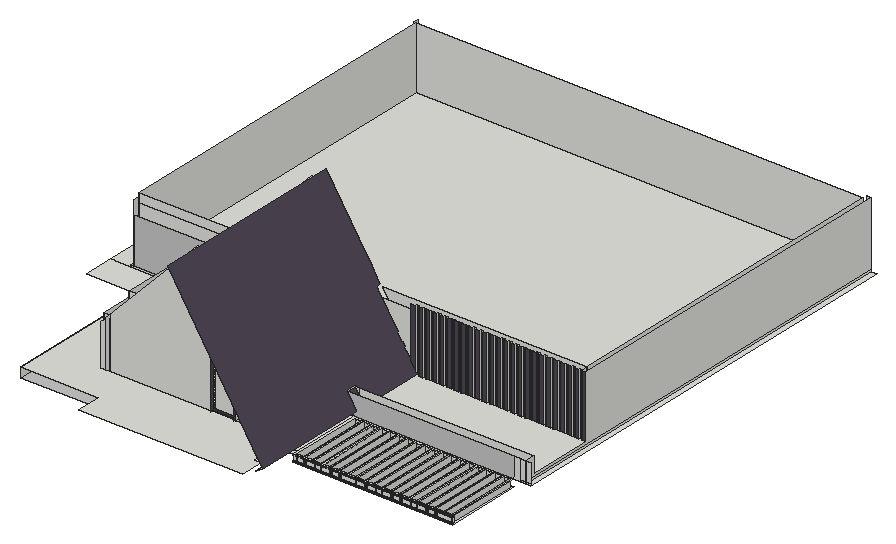
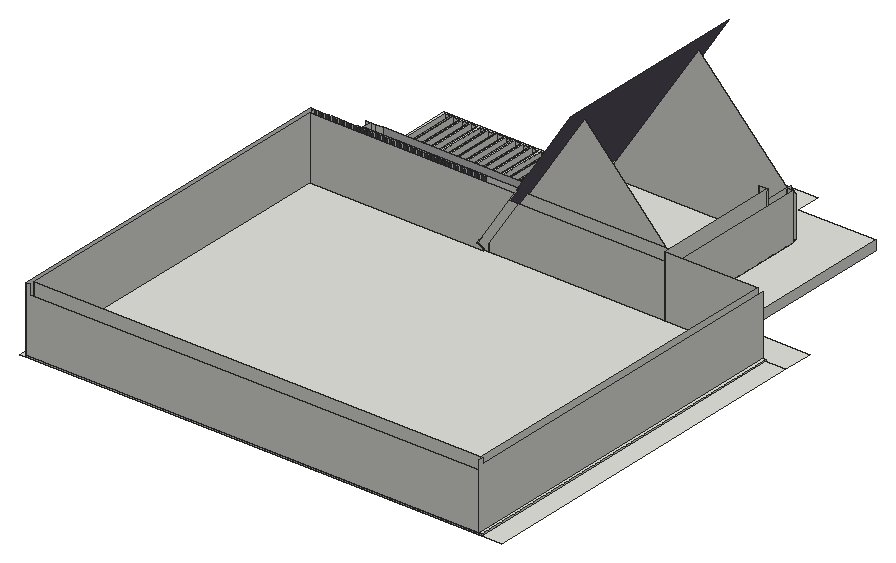
# SketchUp Ruby script. Lengths in inches.
U = 1.inch
M = Sketchup.active_model
def pt(a) = Geom::Point3d.new(a.map { |v| v * U })
def face(e, loops, mat)
  f = e.add_face(loops[0].map { |a| pt(a) })
  loops[1..].each { |l| e.add_face(l.map { |a| pt(a) }).erase! }
  f.material = f.back_material = mat if mat
  f
end
# faces: each face lists its corners as indices into pts; further lists are holes
def faces(e, pts, list, mat = nil) = list.each { |f| face(e, (f[0].is_a?(Array) ? f : [f]).map { |l| l.map { |i| pts[i] } }, mat) }
# xy, xz, yz: faces in a plane at the given z, y or x. An outline is a flat list of corners, or four numbers for a rectangle; further outlines are holes
def ring(l) = l.size == 4 ? [[l[0], l[1]], [l[2], l[1]], [l[2], l[3]], [l[0], l[3]]] : l.each_slice(2).to_a
def flat(e, list, mat, &to3) = list.each { |f| face(e, (f[0].is_a?(Array) ? f : [f]).map { |l| ring(l).map { |u, v| to3.(u, v) } }, mat) }
def xy(e, z, list, mat = nil) = flat(e, list, mat) { |x, y| [x, y, z] }
def xz(e, y, list, mat = nil) = flat(e, list, mat) { |x, z| [x, y, z] }
def yz(e, x, list, mat = nil) = flat(e, list, mat) { |y, z| [x, y, z] }
def lines(e, pts, list) = list.each { |a, b| e.add_line(pt(pts[a]), pt(pts[b])) }
# prism: a flat outline (further loops are holes) pulled along v
def prism(e, loops, v, mat = nil)
  f = face(e, loops, mat); d = Geom::Vector3d.new(v.map { |x| x * U })
  f.pushpull(f.normal.samedirection?(d) ? d.length : -d.length)
end
def box(e, o, s, mat = nil) = prism(e, [[o, [o[0] + s[0], o[1], o[2]], [o[0] + s[0], o[1] + s[1], o[2]], [o[0], o[1] + s[1], o[2]]]], [0, 0, s[2]], mat)
def at(x, y, z, deg = 0) = Geom::Transformation.translation(pt([x, y, z])) * Geom::Transformation.rotation(ORIGIN, Z_AXIS, deg.degrees)
def axes(o, x, y, z) = Geom::Transformation.new([*x, 0, *y, 0, *z, 0, *pt(o).to_a, 1])
def part(name) = M.definitions.add(name)
# library, detail: a bought-in or finely detailed component or shape, given as its bounding box
def library(name, o, s) = part(name).tap { |d| box(d.entities, o, s) }
def detail(e, o, s) = box(e.add_group.entities, o, s)
def put(e, d, t, mat = nil) = e.add_instance(d, t).tap { |i| i.material = mat if mat }
def group(e, t, mat = nil) = e.add_group.tap { |g| g.transformation = t; g.material = mat if mat }.entities
root = M.entities
M.materials.add("[Color M01]").color = [226, 226, 226]
M.materials.add("[Color M02]").color = [198, 198, 198]
M.materials.add("[Color M06]").color = [79, 71, 84]
M.materials.add("[Color M07]").color = [58, 58, 58]
c1 = library("Group\#13",[0,0,0],[3.54,3.54,3.9375])
xy(root,240.47,[[982.37,2357.31,986.75,2413.37],[982.37,2413.37,986.75,2419.01],[986.75,2413.37,997.51,2419.01],[982.37,2419.01,986.75,2443.81],[986.75,2419.01,997.51,2443.81],
  [982.37,2443.81,986.75,2498.31],[986.75,2443.81,997.51,2498.31]])
xy(root,240.88,[[[1205.57,2373.56,1419.96,2475.84],[1408.55,2375.3,1417.24,2472.37],[1396.86,2375.3,1405.55,2472.37],[1385.17,2375.3,1393.86,2472.37],[1373.49,2375.3,1382.17,2472.37],[1361.8,2375.3,1370.49,2472.37],[1350.11,2375.3,1358.8,2472.37],[1338.42,2375.3,1347.11,2472.37],[1326.74,2375.3,1335.42,2472.37],[1315.05,2375.3,1323.74,2472.37],[1303.36,2375.3,1312.05,2472.37],[1291.67,2375.3,1300.36,2472.37],[1279.99,2375.3,1288.67,2472.37],[1268.3,2375.3,1276.99,2472.37],[1256.61,2375.3,1265.3,2472.37],[1244.92,2375.3,1253.61,2472.37],[1233.24,2375.3,1241.92,2472.37],[1221.55,2375.3,1230.24,2472.37],[1209.86,2375.3,1218.55,2472.37]]])
xy(root,242.34,[[1205.57,2373.56,1419.96,2374.81]])
xy(root,249.61,[[1205.57,2373.56,1419.96,2374.81]])
xy(root,251.0625,[[982.37,2357.31,986.75,2413.37],[986.75,2373.56,986.75,2413.37,997.51,2413.37,997.51,2414.32,1083.76,2414.32,1083.76,2373.56],[1083.76,2373.56,1137.16,2414.32],[1137.16,2373.56,1137.16,2414.32,1190.0625,2414.32,1190.0625,2379.76,1205.57,2379.76,1205.57,2373.56],[[1205.57,2373.56,1419.96,2475.84],[1408.55,2375.3,1417.24,2472.37],[1396.86,2375.3,1405.55,2472.37],[1385.17,2375.3,1393.86,2472.37],[1373.49,2375.3,1382.17,2472.37],[1361.8,2375.3,1370.49,2472.37],[1350.11,2375.3,1358.8,2472.37],[1338.42,2375.3,1347.11,2472.37],[1326.74,2375.3,1335.42,2472.37],[1315.05,2375.3,1323.74,2472.37],[1303.36,2375.3,1312.05,2472.37],[1291.67,2375.3,1300.36,2472.37],[1279.99,2375.3,1288.67,2472.37],[1268.3,2375.3,1276.99,2472.37],[1256.61,2375.3,1265.3,2472.37],[1244.92,2375.3,1253.61,2472.37],[1233.24,2375.3,1241.92,2472.37],[1221.55,2375.3,1230.24,2472.37],[1209.86,2375.3,1218.55,2472.37]],
  [1190.0625,2379.76,1205.57,2475.84],[954.51,2413.37,965.32,2414.32],[965.32,2413.37,982.37,2414.32],[982.37,2413.37,997.51,2419.01],[997.51,2414.32,997.51,2584.32,831.14,2584.32,831.14,3047.67,1429.3,3047.67,1429.3,2482.04,1190.0625,2482.04,1190.0625,2414.32],
  [954.51,2419.01,965.32,2498.31],[965.32,2419.01,982.37,2498.31],[982.37,2419.01,982.37,2498.31,965.32,2498.31,965.32,2584.32,997.51,2584.32,997.51,2419.01],[1429.3,2475.84,1429.3,3047.67,831.14,3047.67,831.14,2584.32,954.51,2584.32,954.51,2578.12,943.125,2578.12,943.125,2538.31,881.75,2538.31,881.75,2578.12,824.9375,2578.12,824.9375,3053.87,1435.5,3053.87,1435.5,2475.84],[1435.5,2475.84,1442.5,3053.87],
  [943.125,2498.31,954.51,2578.12],[954.51,2498.31,965.32,2584.32],[797.6875,2538.31,881.75,2578.12],[797.6875,2578.12,824.9375,3053.87]])
xy(root,251.0625,[[881.75,2321.87,881.75,2538.31,943.125,2538.31,943.125,2498.31,954.51,2498.31,954.51,2413.37,982.37,2413.37,982.37,2357.31,986.75,2357.31,986.75,2321.87]],"[Color M02]")
xy(root,253.4375,[[948.3125,2393.06,954.51,2393.06,954.51,2584.32,831.14,2584.32,831.14,3047.67,1429.3,3047.67,1429.3,2475.84,1435.5,2475.84,1435.5,3053.87,828.75,3053.87,828.75,2578.12,881.75,2578.12,881.75,2538.31,948.3125,2538.31],[824.9375,2578.12,828.75,3053.87]])
xy(root,257.0625,[[948.3125,2373.56,954.51,2380.48],[954.51,2373.56,955.23,2380.48],[955.23,2373.56,1190.19,2380.48],[1190.19,2373.56,1196.26,2578.12],[1196.26,2373.56,1205.57,2380.48],
  [946.73,2380.48,954.51,2571.59],[954.51,2380.48,955.23,2571.59],[955.23,2380.48,1190.19,2571.59],[1196.26,2380.48,1205.57,2475.84],[1196.26,2488.81,1435.5,2488.81,1435.5,2576.81,1429.42,2576.81,1429.42,2578.12,1426,2578.12,1426,2576.81,1419.92,2576.81,1419.92,2578.12,1416.5,2578.12,1416.5,2576.81,1410.42,2576.81,1410.42,2578.12,1407,2578.12,1407,2576.81,1400.92,2576.81,1400.92,2578.12,1397.5,2578.12,1397.5,2576.81,1391.42,2576.81,1391.42,2578.12,1388,2578.12,1388,2576.81,1381.92,2576.81,1381.92,2578.12,1378.5,2578.12,1378.5,2576.81,1372.42,2576.81,1372.42,2578.12,1369,2578.12,1369,2576.81,1362.92,2576.81,1362.92,2578.12,1359.5,2578.12,1359.5,2576.81,1353.42,2576.81,1353.42,2578.12,1350,2578.12,1350,2576.81,1343.92,2576.81,1343.92,2578.12,1340.5,2578.12,1340.5,2576.81,1334.42,2576.81,1334.42,2578.12,1331,2578.12,1331,2576.81,1324.92,2576.81,1324.92,2578.12,1321.5,2578.12,1321.5,2576.81,1315.42,2576.81,1315.42,2578.12,1312,2578.12,1312,2576.81,1305.92,2576.81,1305.92,2578.12,1302.5,2578.12,1302.5,2576.81,1296.42,2576.81,1296.42,2578.12,1293,2578.12,1293,2576.81,1286.92,2576.81,1286.92,2578.12,1283.5,2578.12,1283.5,2576.81,1277.42,2576.81,1277.42,2578.12,1274,2578.12,1274,2576.81,1267.92,2576.81,1267.92,2578.12,1264.5,2578.12,1264.5,2576.81,1258.42,2576.81,1258.42,2578.12,1255,2578.12,1255,2576.81,1248.92,2576.81,1248.92,2578.12,1245.5,2578.12,1245.5,2576.81,1239.42,2576.81,1239.42,2578.12,1236,2578.12,1236,2576.81,1229.92,2576.81,1229.92,2578.12,1226.5,2578.12,1226.5,2576.81,1220.42,2576.81,1220.42,2578.12,1217,2578.12,1217,2576.81,1210.92,2576.81,1210.92,2578.12,1196.26,2578.12],
  [948.3125,2571.59,954.51,2578.12],[954.51,2571.59,955.23,2578.12],[955.23,2571.59,1190.19,2578.12],[1210.92,2576.81,1210.92,2578.12,1196.26,2578.12,1196.26,2584.2,1429.42,2584.2,1429.42,2578.12,1426,2578.12,1426,2576.81,1419.92,2576.81,1419.92,2578.12,1416.5,2578.12,1416.5,2576.81,1410.42,2576.81,1410.42,2578.12,1407,2578.12,1407,2576.81,1400.92,2576.81,1400.92,2578.12,1397.5,2578.12,1397.5,2576.81,1391.42,2576.81,1391.42,2578.12,1388,2578.12,1388,2576.81,1381.92,2576.81,1381.92,2578.12,1378.5,2578.12,1378.5,2576.81,1372.42,2576.81,1372.42,2578.12,1369,2578.12,1369,2576.81,1362.92,2576.81,1362.92,2578.12,1359.5,2578.12,1359.5,2576.81,1353.42,2576.81,1353.42,2578.12,1350,2578.12,1350,2576.81,1343.92,2576.81,1343.92,2578.12,1340.5,2578.12,1340.5,2576.81,1334.42,2576.81,1334.42,2578.12,1331,2578.12,1331,2576.81,1324.92,2576.81,1324.92,2578.12,1321.5,2578.12,1321.5,2576.81,1315.42,2576.81,1315.42,2578.12,1312,2578.12,1312,2576.81,1305.92,2576.81,1305.92,2578.12,1302.5,2578.12,1302.5,2576.81,1296.42,2576.81,1296.42,2578.12,1293,2578.12,1293,2576.81,1286.92,2576.81,1286.92,2578.12,1283.5,2578.12,1283.5,2576.81,1277.42,2576.81,1277.42,2578.12,1274,2578.12,1274,2576.81,1267.92,2576.81,1267.92,2578.12,1264.5,2578.12,1264.5,2576.81,1258.42,2576.81,1258.42,2578.12,1255,2578.12,1255,2576.81,1248.92,2576.81,1248.92,2578.12,1245.5,2578.12,1245.5,2576.81,1239.42,2576.81,1239.42,2578.12,1236,2578.12,1236,2576.81,1229.92,2576.81,1229.92,2578.12,1226.5,2578.12,1226.5,2576.81,1220.42,2576.81,1220.42,2578.12,1217,2578.12,1217,2576.81],[955.23,2578.12,1190.19,2584.2],
  [1190.19,2578.12,1196.26,2584.2],[831.01,2584.2,1196.26,2584.2,1196.26,2586.43,1429.42,2586.43,1429.42,3047.79,831.01,3047.79],[1196.26,2584.2,1429.42,2586.43]])
xy(root,263.89,[[[986.75,2289.06,1205.57,2289.06,1205.57,2319.18,1196.26,2319.18,1196.26,2373.56,1129.63,2373.56,1129.63,2371.68,1127.76,2371.68,1127.76,2373.56,1096.79,2373.56,1096.79,2371.68,1095.04,2371.68,1095.04,2373.56,948.3125,2373.56,948.3125,2380.48,946.73,2380.48,946.73,2571.59,948.3125,2571.59,948.3125,2578.12,881.75,2578.12,881.75,2321.87,986.75,2321.87],[949.71,2332.13,1019.02,2332.76]],[1095.04,2373.56,1096.79,2378.12],[1096.79,2373.56,1127.76,2375.74],[1127.76,2373.56,1129.63,2378.12]])
xz(root,2373.56,[[948.3125,263.89,955.23,263.89,955.23,325.17,954.29,324.17,953.84,324.6,952.96,323.67,953.42,323.24,951,320.67,950.54,321.1,949.66,320.17,950.12,319.74,948.77,318.3,948.3125,317.82],[1190.19,263.89,1191.51,263.89,1190.19,265.95],[1191.51,263.89,1191.89,263.89,1190.19,266.53,1190.19,265.95]])
xz(root,2374.81,[[1205.57,242.34,1419.96,249.61]],"[Color M01]")
xz(root,2375.3,[[1209.86,240.88,1218.55,251.0625],[1221.55,240.88,1230.24,251.0625],[1233.24,240.88,1241.92,251.0625],[1244.92,240.88,1253.61,251.0625],[1256.61,240.88,1265.3,251.0625],
  [1268.3,240.88,1276.99,251.0625],[1279.99,240.88,1288.67,251.0625],[1291.67,240.88,1300.36,251.0625],[1303.36,240.88,1312.05,251.0625],[1315.05,240.88,1323.74,251.0625],
  [1326.74,240.88,1335.42,251.0625],[1338.42,240.88,1347.11,251.0625],[1350.11,240.88,1358.8,251.0625],[1361.8,240.88,1370.49,251.0625],[1373.49,240.88,1382.17,251.0625],
  [1385.17,240.88,1393.86,251.0625],[1396.86,240.88,1405.55,251.0625],[1408.55,240.88,1417.24,251.0625]])
xz(root,2375.74,[[1096.79,263.89,1127.76,267.02]],"[Color M06]")
xz(root,2378.12,[[1095.04,263.89,1096.79,412.22],[1127.76,263.89,1129.63,363.92]])
xz(root,2380.48,[[946.73,257.0625,948.3125,258.95],[948.3125,257.0625,955.23,257.0625,955.23,326.08,946.73,326.08,946.73,263.89,948.3125,263.89],[955.23,257.0625,955.23,326.08,1072.29,450.4375,1190.19,266.53,1190.19,257.0625],[946.73,258.95,948.3125,263.89]])
xz(root,2413.37,[[982.37,240.47,986.75,251.0625],[986.75,240.47,997.51,251.0625],[954.51,251.0625,965.32,340.125]])
xz(root,2419.01,[[982.37,240.47,997.51,251.0625]])
xz(root,2472.37,[[1209.86,240.88,1218.55,251.0625],[1221.55,240.88,1230.24,251.0625],[1233.24,240.88,1241.92,251.0625],[1244.92,240.88,1253.61,251.0625],[1256.61,240.88,1265.3,251.0625],
  [1268.3,240.88,1276.99,251.0625],[1279.99,240.88,1288.67,251.0625],[1291.67,240.88,1300.36,251.0625],[1303.36,240.88,1312.05,251.0625],[1315.05,240.88,1323.74,251.0625],
  [1326.74,240.88,1335.42,251.0625],[1338.42,240.88,1347.11,251.0625],[1350.11,240.88,1358.8,251.0625],[1361.8,240.88,1370.49,251.0625],[1373.49,240.88,1382.17,251.0625],
  [1385.17,240.88,1393.86,251.0625],[1396.86,240.88,1405.55,251.0625],[1408.55,240.88,1417.24,251.0625]])
xz(root,2475.84,[[1419.96,251.0625,1429.3,278.1875],[1429.3,251.0625,1435.5,253.4375],[1435.5,251.0625,1442.5,253.4375],[1429.3,253.4375,1435.5,278.1875],[1435.5,253.4375,1442.5,278.1875]])
xz(root,2475.84,[[1205.57,251.0625,1419.96,251.0625,1419.96,278.1875,1196.26,278.1875,1196.26,257.0625,1205.57,257.0625]],"[Color M02]")
xz(root,2488.81,[[1196.26,257.0625,1201.98,278.1875],[1201.98,257.0625,1435.5,278.1875]])
xz(root,2538.31,[[881.75,251.0625,948.3125,253.4375]])
xz(root,2571.59,[[946.73,257.0625,948.3125,258.95],[948.3125,257.0625,948.3125,263.89,946.73,263.89,946.73,326.08,955.23,326.08,955.23,257.0625],[955.23,257.0625,1190.19,257.0625,1190.19,266.53,1072.29,450.4375,977.92,350.1875,968.45,340.125,955.23,326.08],[946.73,258.95,948.3125,263.89]])
xz(root,2576.81,[[1210.92,257.0625,1217,340.125],[1220.42,257.0625,1226.5,340.125],[1229.92,257.0625,1236,340.125],[1239.42,257.0625,1245.5,340.125],[1248.92,257.0625,1255,340.125],
  [1258.42,257.0625,1264.5,340.125],[1267.92,257.0625,1274,340.125],[1277.42,257.0625,1283.5,340.125],[1286.92,257.0625,1293,340.125],[1296.42,257.0625,1302.5,340.125],
  [1305.92,257.0625,1312,340.125],[1315.42,257.0625,1321.5,340.125],[1324.92,257.0625,1331,340.125],[1334.42,257.0625,1340.5,340.125],[1343.92,257.0625,1350,340.125],
  [1353.42,257.0625,1359.5,340.125],[1362.92,257.0625,1369,340.125],[1372.42,257.0625,1378.5,340.125],[1381.92,257.0625,1388,340.125],[1391.42,257.0625,1397.5,340.125],
  [1400.92,257.0625,1407,340.125],[1410.42,257.0625,1416.5,340.125],[1419.92,257.0625,1426,340.125],[1429.42,257.0625,1435.5,340.125],[1207.5,260.03,1207.5,340.125,1201.42,340.125,1201.42,269.51,1201.52,269.35,1205.57,263.03]],"[Color M06]")
xz(root,2578.12,[[824.9375,251.0625,881.75,253.4375],[943.125,251.0625,954.51,251.0625,954.51,257.0625,948.3125,257.0625,948.3125,258.95,943.125,258.95],[1199.5,252.01,1196.26,257.0625,1201.98,257.0625,1203.55,254.61],[1203.55,254.61,1201.98,257.0625,1207.38,257.0625],[955.23,257.0625,1182.42,257.0625,1182.42,278.65,1143.01,340.125,955.23,340.125],
  [1182.42,257.0625,1188.5,257.0625,1188.5,269.17,1182.42,278.65],[1188.5,257.0625,1191.92,257.0625,1191.92,263.83,1190.19,266.53,1188.5,269.17],[1191.92,257.0625,1196.26,257.0625,1191.92,263.83],[1196.26,257.0625,1196.26,265.98,1191.92,272.75,1191.92,263.83],[1196.26,257.0625,1198,257.0625,1198,258.18],
  [1196.26,257.0625,1198,258.18,1198,263.27,1196.26,265.98],[1198,257.0625,1201.42,257.0625,1201.42,257.93,1200.3125,259.66,1198,258.18],[1201.42,257.0625,1201.98,257.0625,1201.42,257.93],[1201.98,257.0625,1207.38,257.0625,1207.5,257.14,1207.5,260.03,1205.57,263.03,1201.42,260.37,1201.42,257.93],[1207.38,257.0625,1207.5,257.0625,1207.5,257.14],
  [1207.5,257.14,1208.8125,257.98,1207.5,260.03],[1201.42,257.93,1201.42,260.37,1200.3125,259.66],[1198,258.18,1200.3125,259.66,1198,263.27],[881.75,258.95,943.125,263.89],[943.125,258.95,948.3125,263.89],
  [1200.3125,259.66,1201.42,260.37,1201.42,269.29,1198,267.09,1198,263.27],[1201.42,260.37,1205.57,263.03,1201.52,269.35,1201.42,269.29],[1198,263.27,1198,267.09,1196.26,265.98],[1191.92,263.83,1191.92,272.75,1188.5,278.09,1188.5,269.17,1190.19,266.53],[943.125,263.89,948.3125,315.25]])
xz(root,2578.12,[[828.75,253.4375,881.75,253.4375,881.75,263.89,943.125,263.89,943.125,315.25,828.75,315.25]],"[Color M02]")
xz(root,2578.12,[[1207.5,257.0625,1210.92,257.0625,1210.92,340.125,1207.5,340.125,1207.5,260.03,1208.8125,257.98,1207.5,257.14],[1217,257.0625,1220.42,340.125],[1226.5,257.0625,1229.92,340.125],[1236,257.0625,1239.42,340.125],[1245.5,257.0625,1248.92,340.125],
  [1255,257.0625,1258.42,340.125],[1264.5,257.0625,1267.92,340.125],[1274,257.0625,1277.42,340.125],[1283.5,257.0625,1286.92,340.125],[1293,257.0625,1296.42,340.125],
  [1302.5,257.0625,1305.92,340.125],[1312,257.0625,1315.42,340.125],[1321.5,257.0625,1324.92,340.125],[1331,257.0625,1334.42,340.125],[1340.5,257.0625,1343.92,340.125],
  [1350,257.0625,1353.42,340.125],[1359.5,257.0625,1362.92,340.125],[1369,257.0625,1372.42,340.125],[1378.5,257.0625,1381.92,340.125],[1388,257.0625,1391.42,340.125],
  [1397.5,257.0625,1400.92,340.125],[1407,257.0625,1410.42,340.125],[1416.5,257.0625,1419.92,340.125],[1426,257.0625,1429.42,340.125]],"[Color M06]")
xz(root,2584.2,[[831.01,257.0625,955.23,328],[955.23,257.0625,955.23,326.08,957.04,328,1150.78,328,1190.19,266.53,1190.19,257.0625],[1190.19,257.0625,1190.19,266.53,1150.78,328,1429.3,328,1429.3,340.125,1429.42,340.125,1429.42,257.0625]])
xz(root,2584.32,[[831.14,251.0625,954.51,253.4375],[831.14,253.4375,954.51,340.125]])
xz(root,2586.43,[[1196.26,257.0625,1200.3125,259.66,1205.57,263.03,1201.52,269.35,1196.26,277.56,1156.15,340.125,1429.42,340.125,1429.42,257.0625]])
xz(root,3047.67,[[831.14,251.0625,1429.3,253.4375],[831.14,253.4375,1429.3,340.125]])
xz(root,3053.87,[[824.9375,251.0625,1435.5,253.4375],[828.75,253.4375,828.75,328,1429.3,328,1429.3,340.125,1435.5,340.125,1435.5,253.4375]])
yz(root,824.9375,[[2578.12,251.0625,3053.87,253.4375]])
yz(root,828.75,[[2578.12,253.4375,2578.12,333.125,3047.67,333.125,3047.67,340.125,3053.87,340.125,3053.87,253.4375]])
yz(root,831.14,[[2584.32,251.0625,3047.67,253.4375],[2584.32,253.4375,3047.67,340.125]])
yz(root,881.75,[[2321.87,251.0625,2321.87,263.89,2578.12,263.89,2578.12,253.4375,2538.31,253.4375,2538.31,251.0625],[2538.31,251.0625,2578.12,253.4375]])
yz(root,946.73,[[2380.48,257.0625,2571.59,258.95],[2380.48,258.95,2571.59,263.89],[2380.48,263.89,2571.59,326.08]])
yz(root,948.3125,[[2373.56,257.0625,2380.48,258.95],[2571.59,257.0625,2578.12,258.95],[2373.56,258.95,2380.48,263.89],[2571.59,258.95,2578.12,263.89]])
yz(root,954.51,[[2413.37,251.0625,2414.32,253.4375],[2414.32,251.0625,2578.12,253.4375],[2578.12,251.0625,2584.32,253.4375],[2413.37,253.4375,2414.32,257.0625],[2414.32,253.4375,2578.12,257.0625],
  [2578.12,253.4375,2584.32,253.4375,2584.32,340.125,2414.32,340.125,2414.32,257.0625,2578.12,257.0625],[2413.37,257.0625,2414.32,340.125]])
yz(root,955.23,[[2373.56,257.0625,2380.48,326.08],[2380.48,257.0625,2571.59,326.08],[2571.59,257.0625,2578.12,326.08],[2578.12,257.0625,2584.2,326.08]])
yz(root,965.32,[[2413.37,251.0625,2414.32,340.125]])
yz(root,982.37,[[2357.31,240.47,2413.37,251.0625],[2413.37,240.47,2419.01,251.0625],[2419.01,240.47,2443.81,251.0625],[2443.81,240.47,2498.31,251.0625]],"[Color M07]")
yz(root,986.75,[[2373.56,240.47,2413.37,251.0625]])
yz(root,997.51,[[2413.37,240.47,2419.01,251.0625]])
yz(root,1095.04,[[2373.56,263.89,2378.12,412.22]])
yz(root,1096.79,[[2375.74,263.89,2378.12,267.02]])
yz(root,1096.79,[[2371.68,263.89,2375.74,263.89,2375.74,267.02,2378.12,267.02,2378.12,267.83,2375.74,267.83,2375.74,270.95,2378.12,270.95,2378.12,271.76,2375.74,271.76,2375.74,274.89,2378.12,274.89,2378.12,275.7,2375.74,275.7,2375.74,278.83,2378.12,278.83,2378.12,279.64,2375.74,279.64,2375.74,282.77,2378.12,282.77,2378.12,283.58,2375.74,283.58,2375.74,286.7,2378.12,286.7,2378.12,287.51,2375.74,287.51,2375.74,290.64,2378.12,290.64,2378.12,291.45,2375.74,291.45,2375.74,294.58,2378.12,294.58,2378.12,295.39,2375.74,295.39,2375.74,298.52,2378.12,298.52,2378.12,299.33,2375.74,299.33,2375.74,302.45,2378.12,302.45,2378.12,303.26,2375.74,303.26,2375.74,306.39,2378.12,306.39,2378.12,307.2,2375.74,307.2,2375.74,310.33,2378.12,310.33,2378.12,311.14,2375.74,311.14,2375.74,314.27,2378.12,314.27,2378.12,315.08,2376.24,315.08,2376.24,318.2,2378.12,318.2,2378.12,319.01,2376.24,319.01,2376.24,322.14,2378.12,322.14,2378.12,322.89,2376.24,322.89,2376.24,326.02,2378.12,326.02,2378.12,326.76,2376.24,326.76,2376.24,329.89,2378.12,329.89,2378.12,330.64,2376.24,330.64,2376.24,333.77,2378.12,333.77,2378.12,334.51,2376.24,334.51,2376.24,337.64,2378.12,337.64,2378.12,338.39,2376.24,338.39,2376.24,341.52,2378.12,341.52,2378.12,341.93,2376.24,341.93,2376.24,345.06,2378.12,345.06,2378.12,346,2376.24,346,2376.24,349.12,2378.12,349.12,2378.12,350.06,2376.24,350.06,2376.24,353.18,2378.12,353.18,2378.12,354.12,2376.24,354.12,2376.24,357.25,2378.12,357.25,2378.12,358.06,2376.24,358.06,2376.24,361.18,2378.12,361.18,2378.12,362,2376.24,362,2376.24,365.12,2378.12,365.12,2378.12,366.25,2376.24,366.25,2376.24,369.37,2378.12,369.37,2378.12,370.5,2376.24,370.5,2376.24,373.62,2378.12,373.62,2378.12,374.75,2376.24,374.75,2376.24,377.87,2378.12,377.87,2378.12,379,2376.24,379,2376.24,382.12,2378.12,382.12,2378.12,383.25,2376.24,383.25,2376.24,386.37,2378.12,386.37,2378.12,387.5,2376.24,387.5,2376.24,390.62,2378.12,390.62,2378.12,391.75,2376.24,391.75,2376.24,394.87,2378.12,394.87,2378.12,396,2376.24,396,2376.24,399.12,2378.12,399.12,2378.12,400.25,2376.24,400.25,2376.24,403.37,2378.12,403.37,2378.12,404.5,2376.24,404.5,2376.24,407.62,2378.12,407.62,2378.12,412.22,2371.68,412.22]],"[Color M06]")
yz(root,1127.76,[[2375.74,263.89,2378.12,267.02]])
yz(root,1127.76,[[2371.68,263.89,2371.68,363.92,2376.24,363.92,2376.24,362,2378.12,362,2378.12,361.18,2376.24,361.18,2376.24,358.06,2378.12,358.06,2378.12,357.25,2376.24,357.25,2376.24,354.12,2378.12,354.12,2378.12,353.18,2376.24,353.18,2376.24,350.06,2378.12,350.06,2378.12,349.12,2376.24,349.12,2376.24,346,2378.12,346,2378.12,345.06,2376.24,345.06,2376.24,341.93,2378.12,341.93,2378.12,341.52,2376.24,341.52,2376.24,338.39,2378.12,338.39,2378.12,337.64,2376.24,337.64,2376.24,334.51,2378.12,334.51,2378.12,333.77,2376.24,333.77,2376.24,330.64,2378.12,330.64,2378.12,329.89,2376.24,329.89,2376.24,326.76,2378.12,326.76,2378.12,326.02,2376.24,326.02,2376.24,322.89,2378.12,322.89,2378.12,322.14,2376.24,322.14,2376.24,319.01,2378.12,319.01,2378.12,318.2,2376.24,318.2,2376.24,315.08,2378.12,315.08,2378.12,314.27,2375.74,314.27,2375.74,311.14,2378.12,311.14,2378.12,310.33,2375.74,310.33,2375.74,307.2,2378.12,307.2,2378.12,306.39,2375.74,306.39,2375.74,303.26,2378.12,303.26,2378.12,302.45,2375.74,302.45,2375.74,299.33,2378.12,299.33,2378.12,298.52,2375.74,298.52,2375.74,295.39,2378.12,295.39,2378.12,294.58,2375.74,294.58,2375.74,291.45,2378.12,291.45,2378.12,290.64,2375.74,290.64,2375.74,287.51,2378.12,287.51,2378.12,286.7,2375.74,286.7,2375.74,283.58,2378.12,283.58,2378.12,282.77,2375.74,282.77,2375.74,279.64,2378.12,279.64,2378.12,278.83,2375.74,278.83,2375.74,275.7,2378.12,275.7,2378.12,274.89,2375.74,274.89,2375.74,271.76,2378.12,271.76,2378.12,270.95,2375.74,270.95,2375.74,267.83,2378.12,267.83,2378.12,267.02,2375.74,267.02,2375.74,263.89]],"[Color M06]")
yz(root,1129.63,[[2373.56,263.89,2378.12,363.92]])
yz(root,1190.19,[[2373.56,257.0625,2380.48,266.53],[2380.48,257.0625,2571.59,266.53],[2571.59,257.0625,2584.2,266.53]])
yz(root,1196.26,[[2475.84,257.0625,2488.81,278.1875]])
yz(root,1207.5,[[2576.81,260.03,2578.12,340.125]])
yz(root,1209.86,[[2375.3,240.88,2472.37,251.0625]])
yz(root,1210.92,[[2576.81,257.0625,2578.12,340.125]])
yz(root,1217,[[2576.81,257.0625,2578.12,340.125]])
yz(root,1218.55,[[2375.3,240.88,2472.37,251.0625]])
yz(root,1220.42,[[2576.81,257.0625,2578.12,340.125]])
yz(root,1221.55,[[2375.3,240.88,2472.37,251.0625]])
yz(root,1226.5,[[2576.81,257.0625,2578.12,340.125]])
yz(root,1229.92,[[2576.81,257.0625,2578.12,340.125]])
yz(root,1230.24,[[2375.3,240.88,2472.37,251.0625]])
yz(root,1233.24,[[2375.3,240.88,2472.37,251.0625]])
yz(root,1236,[[2576.81,257.0625,2578.12,340.125]])
yz(root,1239.42,[[2576.81,257.0625,2578.12,340.125]])
yz(root,1241.92,[[2375.3,240.88,2472.37,251.0625]])
yz(root,1244.92,[[2375.3,240.88,2472.37,251.0625]])
yz(root,1245.5,[[2576.81,257.0625,2578.12,340.125]])
yz(root,1248.92,[[2576.81,257.0625,2578.12,340.125]])
yz(root,1253.61,[[2375.3,240.88,2472.37,251.0625]])
yz(root,1255,[[2576.81,257.0625,2578.12,340.125]])
yz(root,1256.61,[[2375.3,240.88,2472.37,251.0625]])
yz(root,1258.42,[[2576.81,257.0625,2578.12,340.125]])
yz(root,1264.5,[[2576.81,257.0625,2578.12,340.125]])
yz(root,1265.3,[[2375.3,240.88,2472.37,251.0625]])
yz(root,1267.92,[[2576.81,257.0625,2578.12,340.125]])
yz(root,1268.3,[[2375.3,240.88,2472.37,251.0625]])
yz(root,1274,[[2576.81,257.0625,2578.12,340.125]])
yz(root,1276.99,[[2375.3,240.88,2472.37,251.0625]])
yz(root,1277.42,[[2576.81,257.0625,2578.12,340.125]])
yz(root,1279.99,[[2375.3,240.88,2472.37,251.0625]])
yz(root,1283.5,[[2576.81,257.0625,2578.12,340.125]])
yz(root,1286.92,[[2576.81,257.0625,2578.12,340.125]])
yz(root,1288.67,[[2375.3,240.88,2472.37,251.0625]])
yz(root,1291.67,[[2375.3,240.88,2472.37,251.0625]])
yz(root,1293,[[2576.81,257.0625,2578.12,340.125]])
yz(root,1296.42,[[2576.81,257.0625,2578.12,340.125]])
yz(root,1300.36,[[2375.3,240.88,2472.37,251.0625]])
yz(root,1302.5,[[2576.81,257.0625,2578.12,340.125]])
yz(root,1303.36,[[2375.3,240.88,2472.37,251.0625]])
yz(root,1305.92,[[2576.81,257.0625,2578.12,340.125]])
yz(root,1312,[[2576.81,257.0625,2578.12,340.125]])
yz(root,1312.05,[[2375.3,240.88,2472.37,251.0625]])
yz(root,1315.05,[[2375.3,240.88,2472.37,251.0625]])
yz(root,1315.42,[[2576.81,257.0625,2578.12,340.125]])
yz(root,1321.5,[[2576.81,257.0625,2578.12,340.125]])
yz(root,1323.74,[[2375.3,240.88,2472.37,251.0625]])
yz(root,1324.92,[[2576.81,257.0625,2578.12,340.125]])
yz(root,1326.74,[[2375.3,240.88,2472.37,251.0625]])
yz(root,1331,[[2576.81,257.0625,2578.12,340.125]])
yz(root,1334.42,[[2576.81,257.0625,2578.12,340.125]])
yz(root,1335.42,[[2375.3,240.88,2472.37,251.0625]])
yz(root,1338.42,[[2375.3,240.88,2472.37,251.0625]])
yz(root,1340.5,[[2576.81,257.0625,2578.12,340.125]])
yz(root,1343.92,[[2576.81,257.0625,2578.12,340.125]])
yz(root,1347.11,[[2375.3,240.88,2472.37,251.0625]])
yz(root,1350,[[2576.81,257.0625,2578.12,340.125]])
yz(root,1350.11,[[2375.3,240.88,2472.37,251.0625]])
yz(root,1353.42,[[2576.81,257.0625,2578.12,340.125]])
yz(root,1358.8,[[2375.3,240.88,2472.37,251.0625]])
yz(root,1359.5,[[2576.81,257.0625,2578.12,340.125]])
yz(root,1361.8,[[2375.3,240.88,2472.37,251.0625]])
yz(root,1362.92,[[2576.81,257.0625,2578.12,340.125]])
yz(root,1369,[[2576.81,257.0625,2578.12,340.125]])
yz(root,1370.49,[[2375.3,240.88,2472.37,251.0625]])
yz(root,1372.42,[[2576.81,257.0625,2578.12,340.125]])
yz(root,1373.49,[[2375.3,240.88,2472.37,251.0625]])
yz(root,1378.5,[[2576.81,257.0625,2578.12,340.125]])
yz(root,1381.92,[[2576.81,257.0625,2578.12,340.125]])
yz(root,1382.17,[[2375.3,240.88,2472.37,251.0625]])
yz(root,1385.17,[[2375.3,240.88,2472.37,251.0625]])
yz(root,1388,[[2576.81,257.0625,2578.12,340.125]])
yz(root,1391.42,[[2576.81,257.0625,2578.12,340.125]])
yz(root,1393.86,[[2375.3,240.88,2472.37,251.0625]])
yz(root,1396.86,[[2375.3,240.88,2472.37,251.0625]])
yz(root,1397.5,[[2576.81,257.0625,2578.12,340.125]])
yz(root,1400.92,[[2576.81,257.0625,2578.12,340.125]])
yz(root,1405.55,[[2375.3,240.88,2472.37,251.0625]])
yz(root,1407,[[2576.81,257.0625,2578.12,340.125]])
yz(root,1408.55,[[2375.3,240.88,2472.37,251.0625]])
yz(root,1410.42,[[2576.81,257.0625,2578.12,340.125]])
yz(root,1416.5,[[2576.81,257.0625,2578.12,340.125]])
yz(root,1417.24,[[2375.3,240.88,2472.37,251.0625]])
yz(root,1419.92,[[2576.81,257.0625,2578.12,340.125]])
yz(root,1426,[[2576.81,257.0625,2578.12,340.125]])
yz(root,1429.3,[[2475.84,251.0625,2482.04,253.4375],[2482.04,251.0625,3047.67,253.4375]])
yz(root,1429.42,[[2576.81,257.0625,2578.12,340.125],[2578.12,257.0625,2584.2,340.125],[2584.2,257.0625,2586.43,340.125],[2586.43,257.0625,3047.79,340.125]])
yz(root,1435.5,[[2475.84,251.0625,3053.87,253.4375],[2475.84,253.4375,3053.87,253.4375,3053.87,340.125,2576.81,340.125,2576.81,257.0625,2488.81,257.0625,2488.81,278.1875,2475.84,278.1875]])
p = [[1199.5,2571.59,252.01],[1199.5,2578.12,252.01],[1203.55,2578.12,254.61],[1203.55,2319.18,254.61],[1199.5,2319.18,252.01],[1199.5,2373.56,252.01],
  [1199.5,2380.48,252.01],[1199.5,2475.84,252.01],[1199.5,2488.81,252.01],[1196.26,2373.56,257.0625],[1196.26,2380.48,257.0625],[1196.26,2475.84,257.0625],
  [1196.26,2488.81,257.0625],[1196.26,2571.59,257.0625],[1196.26,2578.12,257.0625],[1207.38,2578.12,257.0625],[1207.5,2578.12,257.14],[1208.8125,2578.12,257.98],
  [1208.8125,2319.18,257.98],[1190.19,2380.48,266.53],[1190.19,2373.56,266.53],[1191.89,2373.56,263.89],[1195.05,2373.56,258.95],[1190.19,2571.59,266.53],
  [1190.19,2578.12,266.53],[1191.92,2578.12,263.83],[1198,2578.12,258.18],[1200.3125,2578.12,259.66],[1200.3125,2586.43,259.66],[1196.26,2586.43,257.0625],
  [1196.26,2584.2,257.0625],[1081.6,2578.12,456.41],[1081.6,2319.18,456.41],[1205.03,2319.18,263.89],[1205.57,2319.18,263.03],[1207.5,2578.12,260.03],
  [1207.5,2576.81,260.03],[1205.57,2576.81,263.03],[1201.52,2576.81,269.35],[1201.42,2576.81,269.51],[1201.42,2578.12,269.51],[1198,2578.12,274.85],
  [1198,2576.81,274.85],[1196.26,2576.81,277.56],[1191.92,2576.81,284.33],[1191.92,2578.12,284.33],[1188.5,2578.12,289.67],[1188.5,2576.81,289.67],
  [1182.42,2576.81,299.15],[1182.42,2578.12,299.15],[1156.15,2578.12,340.125],[1153.99,2578.12,343.5],[1153.99,2584.2,343.5],[1149.7,2584.2,350.1875],
  [1138.08,2584.2,368.3125],[1136.41,2584.2,370.91],[1081.6,2584.2,456.41],[1201.42,2578.12,260.37],[1205.57,2578.12,263.03],[1205.57,2586.43,263.03],
  [1201.52,2578.12,269.35],[1201.52,2586.43,269.35],[948.3125,2413.37,240.47],[954.51,2413.37,240.47],[964.5,2498.31,240.47],[964.5,2538.31,240.47],
  [954.51,2414.32,240.47],[948.3125,2393.06,251.0625],[948.3125,2393.06,253.4375],[1195.98,2488.81,257.0625]]
faces(root,p,[[0,1,2,3,4,5,6,7,8],[9,10,6,5],[10,11,7,6],[11,12,8,7],[12,13,0,8],[13,14,1,0],[3,2,15,16,17,18],[10,19,20,21,22,9],
  [19,23,13,12,11,10],[13,23,24,25,14],[14,26,27,28,29,30],[27,57,58,59,28],[35,58,37,36],[58,60,38,37],[58,60,61,59]])
faces(root,p,[[31,32,33,34,18,17,35,36,37,38,39,40,41,42,43,44,45,46,47,48,49,50,51,52,53,54,55,56]],"[Color M06]")
lines(root,p,[[62,63],[64,65],[63,66],[67,68],[12,69]])
put(root,c1,axes([897.3,2428.99,258.17],[-1.5535,0,0],[0,2.39,0],[0,0,-3.63878]))
